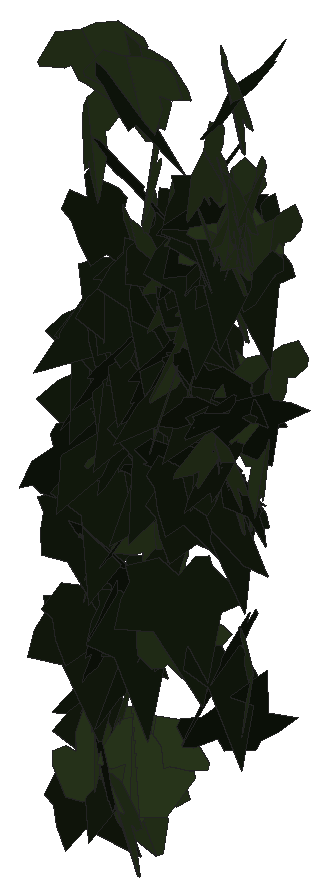
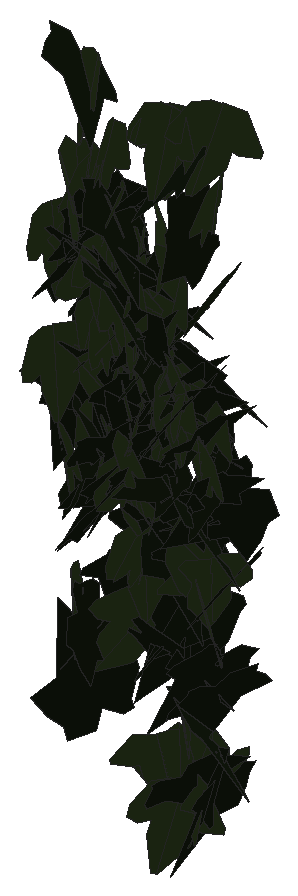
# SketchUp Ruby script. Lengths in inches.
U = 1.inch
M = Sketchup.active_model
def pt(a) = Geom::Point3d.new(a.map { |v| v * U })
def face(e, loops, mat)
  f = e.add_face(loops[0].map { |a| pt(a) })
  loops[1..].each { |l| e.add_face(l.map { |a| pt(a) }).erase! }
  f.material = f.back_material = mat if mat
  f
end
# faces: each face lists its corners as indices into pts; further lists are holes
def faces(e, pts, list, mat = nil) = list.each { |f| face(e, (f[0].is_a?(Array) ? f : [f]).map { |l| l.map { |i| pts[i] } }, mat) }
# xy, xz, yz: faces in a plane at the given z, y or x. An outline is a flat list of corners, or four numbers for a rectangle; further outlines are holes
def ring(l) = l.size == 4 ? [[l[0], l[1]], [l[2], l[1]], [l[2], l[3]], [l[0], l[3]]] : l.each_slice(2).to_a
def flat(e, list, mat, &to3) = list.each { |f| face(e, (f[0].is_a?(Array) ? f : [f]).map { |l| ring(l).map { |u, v| to3.(u, v) } }, mat) }
def xy(e, z, list, mat = nil) = flat(e, list, mat) { |x, y| [x, y, z] }
def xz(e, y, list, mat = nil) = flat(e, list, mat) { |x, z| [x, y, z] }
def yz(e, x, list, mat = nil) = flat(e, list, mat) { |y, z| [x, y, z] }
def lines(e, pts, list) = list.each { |a, b| e.add_line(pt(pts[a]), pt(pts[b])) }
# prism: a flat outline (further loops are holes) pulled along v
def prism(e, loops, v, mat = nil)
  f = face(e, loops, mat); d = Geom::Vector3d.new(v.map { |x| x * U })
  f.pushpull(f.normal.samedirection?(d) ? d.length : -d.length)
end
def box(e, o, s, mat = nil) = prism(e, [[o, [o[0] + s[0], o[1], o[2]], [o[0] + s[0], o[1] + s[1], o[2]], [o[0], o[1] + s[1], o[2]]]], [0, 0, s[2]], mat)
def at(x, y, z, deg = 0) = Geom::Transformation.translation(pt([x, y, z])) * Geom::Transformation.rotation(ORIGIN, Z_AXIS, deg.degrees)
def axes(o, x, y, z) = Geom::Transformation.new([*x, 0, *y, 0, *z, 0, *pt(o).to_a, 1])
def part(name) = M.definitions.add(name)
# library, detail: a bought-in or finely detailed component or shape, given as its bounding box
def library(name, o, s) = part(name).tap { |d| box(d.entities, o, s) }
def detail(e, o, s) = box(e.add_group.entities, o, s)
def put(e, d, t, mat = nil) = e.add_instance(d, t).tap { |i| i.material = mat if mat }
def group(e, t, mat = nil) = e.add_group.tap { |g| g.transformation = t; g.material = mat if mat }.entities
root = M.entities
M.materials.add("efeu1").color = [18, 25, 13]
M.materials.add("efeu2").color = [43, 57, 29]
c1 = part("ivyleaf_10")
p = [[0,0.5,-0.03],[-0.0625,2.02,-0.43],[-0.19,2.01,-0.46],[-0.54,1.05,-0.29],[-0.52,0.625,-0.18],[-0.83,0.76,-0.28],
  [-1.16,0.64,-0.33],[-1.15,0.33,-0.24],[-0.77,-0.39,0.02],[-0.3,-0.51,0.16],[0.04,-0.48,0.23],[-0.02,2.01,-0.4375],
  [-0.06,2.01,-0.43],[0.04,-0.49,0.23],[0.67,-0.49,0.14],[1.38,0.36,-0.2],[1.375,0.51,-0.24],[0.81,0.65,-0.19],
  [0.62,0.59,-0.15],[0.6,1.09,-0.28],[0.5,1.23,-0.31]]
faces(c1.entities,p,[[0,1,2,3,4,5,6,7,8,9,10],[11,12,0,13,14,15,16,17,18,19,20]],"efeu2")
c2 = part("ivyleaf_9")
p = [[1.54,2.16,1.25],[1.36,2.04,1.19],[-0.21,0.99,0.68],[-0.71,1.11,0.82],[-0.85,0.86,0.67],[-0.8,0.17,0.21],
  [-0.9,-0.01,0.1],[-0.67,-0.16,-0.02],[-0.08,-0.08,-0.05],[-0.03,-0.6,-0.4],[0.65,-0.88,-0.66],[0.83,-0.6,-0.49],
  [1.29,-0.42,-0.43],[1.8125,-0.07,-0.26],[1.21,0.44,0.15]]
faces(c2.entities,p,[[0,1,2,3,4,5,6,7,8,9,10,11,12,13,14]],"efeu1")
put(root,c1,axes([35.58,224.02,227.09],[0.29237,0.40468,-0.02738],[-0.03311,-0.00983,-0.49881],[-0.40425,0.29349,0.02105]))
put(root,c2,axes([35.62,223.26,227.93],[-0.05786,0.17102,-0.46627],[-0.11673,0.45159,0.18012],[0.48273,0.12969,-0.01233]))
put(root,c2,axes([35.55,223.95,225.33],[-0.05286,-0.48245,-0.12019],[0.02829,0.11775,-0.48511],[0.49639,-0.05808,0.01485]))
put(root,c2,axes([35.56,223.9,225.74],[0.13724,-0.28703,-0.38572],[-0.033,0.39455,-0.30535],[0.47966,0.10927,0.08935]))
put(root,c2,axes([35.52,223.72,226.78],[0.18225,-0.4637,-0.04201],[-0.00116,0.04466,-0.498],[0.4656,0.18162,0.0152]))
put(root,c2,axes([35.77,224.11,228.19],[-0.27093,-0.41505,0.06578],[-0.02562,-0.06181,-0.4955],[0.41945,-0.27187,0.01223]))
put(root,c1,axes([35.79,223.89,226.62],[0.25583,-0.42854,-0.03],[-0.02347,0.02092,-0.49901],[0.42895,0.25674,-0.00942]))
put(root,c2,axes([36.06,223.89,224.85],[-0.37906,0.31936,0.06574],[-0.05065,0.04192,-0.49566],[-0.3221,-0.38243,0.00057]))
put(root,c1,axes([35.63,224.11,228.86],[0.39028,-0.27171,0.15447],[0.15909,-0.04,-0.47232],[0.26903,0.41782,0.05523]))
put(root,c2,axes([35.77,224.13,229.02],[-0.16658,-0.44457,0.15689],[-0.00294,-0.16541,-0.47184],[0.47143,-0.15812,0.05249]))
put(root,c1,axes([35.89,224.18,227.45],[0.05126,-0.38923,0.30963],[0.01954,-0.30946,-0.39224],[0.49698,0.05231,-0.01651]))
put(root,c2,axes([35.58,223.96,228.3],[0.39911,-0.29966,0.03024],[0.02287,-0.01991,-0.49908],[0.30032,0.39976,-0.00218]))
put(root,c2,axes([36.14,223.89,228],[-0.37119,0.33499,-0.00087],[0.00466,0.00386,-0.49996],[-0.33496,-0.37117,-0.00599]))
put(root,c1,axes([35.92,223.51,223.5625],[0.05534,0.47495,-0.14615],[0.01798,0.14504,0.47816],[0.4966,-0.05818,-0.00102]))
put(root,c2,axes([35.8,223.4,223.62],[0.20539,-0.25517,-0.37776],[-0.19588,0.32473,-0.32585],[0.41164,0.28185,0.03342]))
put(root,c2,axes([36.12,223.52,223.48],[0.03768,-0.18079,0.46464],[-0.13901,0.44368,0.18391],[-0.47881,-0.14304,-0.01683]))
put(root,c2,axes([35.67,223.64,226.58],[0.49636,-0.06024,-0.00054],[-0.0005,0.0004,-0.5],[0.06024,0.49636,0.00034]))
put(root,c2,axes([35.72,223.74,230.99],[0.33858,-0.30268,-0.20917],[-0.08982,0.20766,-0.44588],[0.35679,0.33951,0.08624]))
put(root,c1,axes([35.95,223.49,232.27],[-0.16057,0.47346,-0.00721],[-0.05721,-0.02695,-0.49598],[-0.47005,-0.15846,0.06283]))
put(root,c1,axes([35.95,223.45,233.33],[-0.39805,-0.26984,-0.1369],[0.10745,0.08542,-0.48079],[0.28286,-0.41217,-0.01002]))
put(root,c2,axes([35.92,224.15,223.98],[-0.18209,-0.46377,0.04201],[-0.01122,-0.04072,-0.49821],[0.46553,-0.18238,0.00442]))
put(root,c1,axes([35.91,223.71,229.2],[-0.44819,0.07153,-0.20979],[0.16833,-0.19802,-0.42714],[-0.14419,-0.45351,0.15342]))
put(root,c2,axes([36.29,223.7,229.89],[-0.49647,0.0445,0.03924],[-0.04067,-0.01453,-0.49813],[-0.04319,-0.4978,0.01804]))
put(root,c2,axes([36.11,223.33,225.42],[0.0384,0.13118,0.48096],[0.10577,0.46925,-0.13643],[-0.48717,0.11222,0.00829]))
put(root,c1,axes([36.0625,223.89,228.92],[0.42004,-0.27121,0.00338],[0.00367,-0.00054,-0.49999],[0.27121,0.42005,0.00154]))
put(root,c2,axes([36.0625,223.96,227.27],[-0.19865,-0.45824,0.02356],[0.00015,-0.02574,-0.49934],[0.45884,-0.19838,0.01036]))
put(root,c2,axes([35.91,223.99,229.49],[0.2478,-0.40938,-0.14493],[-0.02852,0.15117,-0.47575],[0.43334,0.24405,0.05157]))
put(root,c2,axes([36.1,224.05,229.39],[-0.27162,-0.41581,-0.05765],[0.05547,0.03251,-0.49585],[0.41611,-0.27576,0.02847]))
put(root,c1,axes([36.2,224.04,229.55],[0.03067,-0.49744,-0.04014],[-0.00841,0.03969,-0.49835],[0.49899,0.03124,-0.00593]))
put(root,c2,axes([36.06,223.65,226.17],[0.47634,0.14014,-0.05885],[-0.05704,-0.01461,-0.49652],[-0.14089,0.47974,0.00206]))
put(root,c1,axes([36.17,224.06,229.56],[-0.37768,0.30504,-0.11962],[0.09173,-0.07681,-0.48548],[-0.31456,-0.38865,0.00206]))
put(root,c1,axes([36.1875,224.09,228.625],[-0.34095,0.26355,-0.25357],[0.05987,-0.30177,-0.39415],[-0.36079,-0.29913,0.17421]))
put(root,c1,axes([36.17,223.65,223.41],[-0.37625,0.30123,-0.13301],[0.09571,-0.0932,-0.48182],[-0.31508,-0.38804,0.01247]))
put(root,c2,axes([36.57,224.09,225.79],[-0.47696,0.09027,0.11983],[-0.11601,0.0313,-0.48535],[-0.09513,-0.49079,-0.00891]))
put(root,c2,axes([36.4375,223.67,229.39],[-0.23732,0.32208,-0.29991],[0.07653,-0.30534,-0.38847],[-0.43339,-0.23029,0.09563]))
put(root,c1,axes([36.27,223.85,223.38],[-0.41164,-0.26234,-0.1083],[0.0914,0.0581,-0.48813],[0.26869,-0.42167,0.00012]))
put(root,c1,axes([36.3125,223.95,229.42],[-0.48671,0.11208,-0.0235],[0.01633,-0.0336,-0.4986],[-0.11335,-0.48612,0.02905]))
put(root,c2,axes([35.97,224.09,228.53],[0.3933,-0.29686,0.08477],[0.0928,-0.01726,-0.49101],[0.29445,0.40197,0.04152]))
put(root,c1,axes([36.37,223.69,225.0625],[0.22934,-0.41286,-0.16416],[-0.06896,0.14942,-0.47214],[0.43892,0.2392,0.0116]))
put(root,c2,axes([36.04,223.63,231.78],[0.4826,-0.13075,-0.00208],[-0.002,0.00055,-0.5],[0.13075,0.4826,0]))
put(root,c2,axes([36.18,224.05,229.5625],[-0.0649,-0.48448,0.10519],[0.00906,-0.10723,-0.48828],[0.49569,-0.06147,0.02269]))
put(root,c2,axes([36.5,223.72,227.14],[-0.20804,0.44959,-0.06772],[0.03901,-0.05654,-0.49526],[-0.45299,-0.21135,-0.01155]))
put(root,c1,axes([36.34,224,229.9],[0.38906,-0.31187,-0.03698],[-0.0339,0.01683,-0.49857],[0.31222,0.39045,-0.00805]))
put(root,c2,axes([36.54,223.83,229.79],[-0.32308,0.29798,-0.23838],[0.07678,-0.25519,-0.42306],[-0.37379,-0.30997,0.11914]))
put(root,c2,axes([36.06,224.11,228.14],[-0.12738,-0.13552,-0.46412],[0.42801,0.19164,-0.17343],[0.22489,-0.44149,0.06719]))
put(root,c2,axes([36.37,224.04,228.94],[-0.20956,-0.43569,0.1275],[-0.05807,-0.11355,-0.48346],[0.45024,-0.21743,-0.00301]))
put(root,c1,axes([36.4375,223.73,230.8],[-0.43674,0.24233,0.02316],[-0.02449,0.00359,-0.49939],[-0.2422,-0.43734,0.00874]))
put(root,c2,axes([36.21,223.53,232.91],[0.41361,-0.24548,-0.13664],[-0.09597,0.1051,-0.47932],[0.26404,0.42272,0.03982]))
put(root,c1,axes([36.46,223.86,229.67],[-0.25974,0.42724,-0.00167],[-0.00058,-0.0023,-0.49999],[-0.42724,-0.25973,0.00169]))
put(root,c1,axes([36.65,223.66,231.31],[0.2073,-0.201,0.4082],[-0.29786,0.27914,0.28872],[-0.34395,-0.36288,-0.00401]))
put(root,c1,axes([36.54,223.51,233.11],[-0.48633,-0.11349,-0.02454],[0.02499,0.0009,-0.49937],[0.11339,-0.48695,0.0048]))
put(root,c1,axes([36.52,223.64,223.51],[0.47654,0.12824,0.08042],[-0.0778,-0.02034,0.49349],[0.12984,-0.48285,0.00057]))
put(root,c1,axes([36.59,223.71,233.18],[-0.48976,0.08982,0.04543],[-0.0424,0.02058,-0.49777],[-0.09129,-0.49144,-0.01254]))
put(root,c2,axes([36.36,223.77,225.7],[0.07903,-0.4934,0.01768],[0.00109,-0.01774,-0.49968],[0.49371,0.07902,-0.00173]))
put(root,c1,axes([36.51,223.88,224.125],[0.38238,0.31526,-0.06629],[-0.04591,-0.04851,-0.49552],[-0.31887,0.38504,-0.00814]))
put(root,c2,axes([36.58,224.01,227.39],[-0.329,-0.17717,-0.33222],[0.29674,0.14955,-0.37361],[0.23175,-0.443,0.00674]))
put(root,c2,axes([36.58,224,230.21],[-0.07296,-0.49252,0.04584],[-0.00488,-0.04562,-0.49789],[0.49462,-0.0731,0.00185]))
put(root,c1,axes([36.78,223.89,227.01],[-0.24818,-0.43402,-0.00605],[0.00096,0.00643,-0.49996],[0.43406,-0.24817,-0.00236]))
put(root,c1,axes([36.65,224.04,227.2],[-0.09472,0.48571,-0.07152],[0.00825,-0.07126,-0.49483],[-0.49088,-0.09492,0.00549]))
put(root,c1,axes([36.97,223.96,228],[-0.43812,-0.12079,0.20847],[-0.1914,-0.08828,-0.4534],[0.14633,-0.47709,0.03111]))
put(root,c1,axes([36.82,224,230.1875],[0.1362,-0.47829,-0.05184],[-0.00165,0.05342,-0.49714],[0.48109,0.13559,0.01297]))
put(root,c2,axes([36.53,223.98,229.96],[0.23357,-0.43868,0.05482],[0.03066,-0.04578,-0.49695],[0.44103,0.23551,0.00552]))
put(root,c1,axes([36.74,224.03,229.15],[-0.25012,0.41202,-0.13298],[0.05637,-0.12128,-0.48178],[-0.42926,-0.256,0.01422]))
put(root,c2,axes([36.67,224.01,229.44],[-0.14992,-0.38232,-0.28522],[0.09773,0.26802,-0.41063],[0.46688,-0.17887,-0.00563]))
put(root,c2,axes([37.19,223.75,230.92],[-0.44642,0.14682,0.17075],[-0.16095,0.05713,-0.46993],[-0.1575,-0.47453,-0.00375]))
put(root,c2,axes([36.82,223.95,228.2],[-0.15141,-0.45532,0.14056],[-0.05104,-0.13114,-0.47979],[0.47378,-0.15964,-0.00677]))
put(root,c2,axes([36.68,224.0625,230.05],[-0.22968,0.17887,0.40651],[0.29396,-0.28183,0.2901],[0.33291,0.37226,0.0243]))
put(root,c2,axes([37.03,223.77,229.49],[-0.16845,0.34759,-0.3175],[0.0737,-0.31358,-0.38241],[-0.46497,-0.17563,0.05441]))
put(root,c1,axes([36.92,223.69,229.1],[0.30462,-0.39646,-0.00485],[-0.00454,0.00262,-0.49997],[0.39647,0.30465,-0.00201]))
put(root,c1,axes([36.95,223.9,230.58],[0.34544,-0.30018,-0.2014],[-0.03595,0.24866,-0.43229],[0.35969,0.31314,0.15021]))
put(root,c1,axes([37.05,223.61,231.1],[0.12911,-0.19025,-0.444],[-0.08887,0.44238,-0.2154],[0.4748,0.13453,0.08042]))
put(root,c2,axes([37.15,223.81,228.17],[-0.47895,-0.14353,-0.00297],[0.00276,0.00116,-0.49999],[0.14353,-0.47896,-0.00032]))
put(root,c1,axes([37.1,223.91,230.66],[-0.06939,-0.49515,-0.00285],[0.00246,0.00254,-0.49999],[0.49516,-0.0694,0.00209]))
put(root,c1,axes([37.09,223.98,229.39],[0.30238,-0.39731,-0.02657],[0.00626,0.0381,-0.49851],[0.39815,0.30115,0.02802]))
put(root,c2,axes([37.32,223.76,229.4],[-0.49271,0.0772,-0.03581],[0.02919,-0.04429,-0.49718],[-0.07993,-0.49202,0.03914]))
put(root,c1,axes([37.11,224.07,228.5],[0.43254,-0.24444,-0.05617],[-0.04311,0.03786,-0.4967],[0.24708,0.43453,0.01167]))
put(root,c1,axes([37.48,223.94,230.7],[0.1,-0.00213,-0.48989],[-0.47903,0.10431,-0.09824],[0.10262,0.48899,0.01882]))
put(root,c1,axes([37.12,223.86,229.68],[-0.06424,0.2198,-0.44448],[-0.04657,-0.44889,-0.21525],[-0.49366,0.01374,0.07815]))
put(root,c2,axes([37.1,224.22,228.61],[-0.1929,-0.46088,-0.01954],[0.00408,0.01948,-0.4996],[0.46127,-0.19291,-0.00375]))
put(root,c2,axes([36.87,223.45,228.0625],[0.43155,0.13812,0.2114],[0.20015,0.06812,-0.4531],[-0.15397,0.47569,0.0035]))
put(root,c1,axes([37.02,223.64,225.76],[-0.39551,-0.13025,-0.27677],[0.26125,0.09149,-0.41639],[0.15912,-0.47399,-0.00432]))
put(root,c2,axes([37.45,223.78,230.84],[-0.20694,0.42813,0.15455],[-0.11063,0.11737,-0.47327],[-0.44152,-0.23007,0.04615]))
put(root,c2,axes([36.91,223.98,230.34],[0.26968,-0.40357,-0.12002],[0.00341,0.14462,-0.47862],[0.42102,0.25733,0.08075]))
put(root,c2,axes([37.4375,223.74,231.76],[-0.19402,0.45843,0.04686],[-0.01204,0.04579,-0.49775],[-0.46066,-0.19428,-0.00673]))
put(root,c1,axes([37.25,224.04,230.16],[0.0101,-0.49814,0.04194],[0.02442,-0.04141,-0.49768],[0.4993,0.0121,0.02349]))
put(root,c1,axes([37.3,223.99,231.17],[-0.18222,-0.45916,-0.07725],[0.0256,0.07295,-0.49399],[0.46491,-0.18398,-0.00308]))
put(root,c2,axes([37.12,223.62,226.53],[-0.1366,-0.40483,-0.25971],[0.12518,0.23076,-0.42554],[0.4644,-0.18128,0.03831]))
put(root,c2,axes([37.16,223.53,228.0625],[0.26816,-0.33308,-0.25912],[-0.15018,0.2116,-0.4274],[0.39438,0.30706,0.01344]))
put(root,c2,axes([37.66,223.9,230.95],[-0.39816,0.28226,0.10863],[-0.13328,-0.00255,-0.4819],[-0.27149,-0.4127,0.07727]))
put(root,c1,axes([37.36,224.01,230.82],[-0.35587,-0.33298,-0.1117],[0.09981,0.05658,-0.48666],[0.33674,-0.36867,0.0262]))
put(root,c2,axes([37.23,223.66,227.78],[0.17761,-0.29381,-0.36349],[-0.05966,0.37142,-0.32937],[0.46357,0.16037,0.09688]))
put(root,c2,axes([37.3,223.94,230.75],[-0.06337,-0.49571,0.01614],[-0.00013,-0.01626,-0.49974],[0.49597,-0.06334,0.00193]))
put(root,c1,axes([37.52,223.6,231.13],[-0.49945,0.02198,0.00827],[-0.00824,0.00101,-0.49993],[-0.022,-0.49952,-0.00064]))
put(root,c2,axes([37.29,224.22,227.51],[0.11508,-0.48655,0.00516],[0.01053,-0.00281,-0.49988],[0.48646,0.11517,0.0096]))
put(root,c1,axes([37.85,223.83,229.16],[-0.24068,0.15229,0.41095],[-0.43777,-0.10572,-0.21721],[0.02074,-0.46436,0.18423]))
put(root,c1,axes([37.53,223.56,231.64],[-0.28413,0.40149,0.08986],[-0.03864,0.08269,-0.4916],[-0.4096,-0.2863,-0.01596]))
put(root,c2,axes([37.7,223.61,231.62],[-0.04625,0.35204,-0.35203],[0.01935,-0.35201,-0.35456],[-0.49748,-0.04642,0.01893]))
put(root,c1,axes([37.65,223.75,228.53],[-0.03744,-0.49814,-0.02142],[-0.00234,0.02165,-0.49953],[0.49859,-0.0373,-0.00396]))
put(root,c2,axes([37.73,223.93,229.49],[-0.48219,-0.11153,-0.07112],[0.07741,-0.01995,-0.49357],[0.10725,-0.487,0.0365]))
put(root,c2,axes([37.61,224.17,225.78],[-0.26166,0.10512,-0.4129],[0.30262,-0.29524,-0.26694],[-0.29993,-0.38959,0.09089]))
put(root,c2,axes([37.43,223.84,231.55],[0.06888,-0.49417,-0.03249],[-0.00856,0.0316,-0.49893],[0.49516,0.06929,-0.00411]))
put(root,c2,axes([37.71,223.45,229.55],[0.32441,0.18972,-0.3298],[-0.2964,-0.14573,-0.37538],[-0.23855,0.43906,0.01791]))
put(root,c1,axes([37.57,223.82,230.86],[-0.37647,0.29815,-0.1392],[0.11393,-0.08032,-0.48017],[-0.30869,-0.39326,-0.00746]))
put(root,c2,axes([37.77,223.51,229.09],[0.20021,0.40156,-0.22061],[-0.1192,-0.18681,-0.44821],[-0.44239,0.23206,0.02093]))
put(root,c2,axes([37.86,223.7,228.56],[-0.40573,0.25505,-0.14259],[0.10743,-0.09669,-0.47865],[-0.27173,-0.41905,0.02366]))
put(root,c2,axes([37.46,223.96,224.45],[0.37467,0.31362,0.10613],[-0.08136,-0.06814,0.48861],[0.32093,-0.38341,-0.00003]))
put(root,c1,axes([37.72,223.62,231.625],[0.39298,-0.29886,-0.07904],[-0.05408,0.05941,-0.4935],[0.30437,0.39643,0.01436]))
put(root,c2,axes([38.02,224.03,231.08],[-0.47433,0.09861,0.12364],[-0.12774,-0.00846,-0.48333],[-0.09323,-0.49011,0.03322]))
put(root,c1,axes([37.72,223.37,232.42],[0.10686,-0.39465,-0.28781],[0.05457,0.30242,-0.39442],[0.48539,0.05288,0.10771]))
put(root,c2,axes([37.52,223.98,225.51],[0.11535,-0.47063,0.1233],[0.05238,-0.11397,-0.48401],[0.48369,0.12457,0.02301]))
put(root,c1,axes([37.74,223.64,228.4375],[-0.38959,0.30678,-0.06409],[0.04796,-0.04268,-0.49586],[-0.30971,-0.39251,0.00383]))
put(root,c1,axes([37.74,223.71,231.34],[0.28351,0.40573,-0.07072],[-0.03294,-0.06324,-0.49489],[-0.41053,0.28527,-0.00913]))
put(root,c2,axes([37.55,224.14,227.85],[0.32777,-0.21206,-0.3124],[0.27251,-0.15349,0.3901],[-0.26135,-0.42599,0.01496]))
put(root,c2,axes([37.71,223.87,231.3],[-0.07157,-0.4948,0.00737],[0.00179,-0.00771,-0.49994],[0.49485,-0.07153,0.00288]))
put(root,c1,axes([37.89,223.83,231.65],[0.14076,-0.47906,0.02618],[0.01083,-0.02411,-0.4993],[0.47965,0.14113,0.00359]))
put(root,c1,axes([37.92,223.57,233.45],[-0.38263,0.31614,0.06046],[-0.06525,0.01578,-0.49547],[-0.31518,-0.38705,0.02918]))
put(root,c1,axes([37.94,223.55,232.03],[-0.40412,0.29425,-0.01039],[0.00905,-0.00522,-0.49989],[-0.29429,-0.40422,-0.00111]))
put(root,c2,axes([37.76,224.05,230.98],[0.10081,-0.48599,-0.06041],[-0.00441,0.06078,-0.49627],[0.48971,0.10059,0.00797]))
put(root,c1,axes([37.92,224.12,228.3],[0.37423,-0.33132,0.01353],[0.04676,0.03254,-0.49674],[0.32828,0.37306,0.05534]))
put(root,c2,axes([37.99,223.49,229.08],[0.27616,0.41559,-0.03193],[-0.02011,-0.02498,-0.49897],[-0.41633,0.27688,0.00292]))
put(root,c1,axes([37.99,223.62,232],[-0.15837,0.47417,-0.00888],[-0.05465,-0.02755,-0.49624],[-0.4711,-0.15621,0.06056]))
put(root,c2,axes([38.27,223.34,233.45],[-0.08416,0.45069,0.19949],[-0.08596,0.18585,-0.45615],[-0.48531,-0.11108,0.0462]))
put(root,c1,axes([38.2,223.53,225.72],[0.18283,-0.2291,-0.40508],[-0.16454,0.37528,-0.28651],[0.43532,0.23806,0.06183]))
put(root,c1,axes([38.12,224.05,229.55],[-0.16578,-0.47093,-0.02726],[0.00887,0.02577,-0.49926],[0.47163,-0.16602,-0.00019]))
put(root,c1,axes([38.17,224,231.34],[-0.07856,-0.49229,-0.03843],[0.00148,0.03868,-0.4985],[0.49379,-0.07844,-0.00462]))
put(root,c1,axes([38.14,223.77,232.05],[0.25431,-0.42807,0.04563],[0.02475,-0.03837,-0.49791],[0.42979,0.2555,0.00168]))
